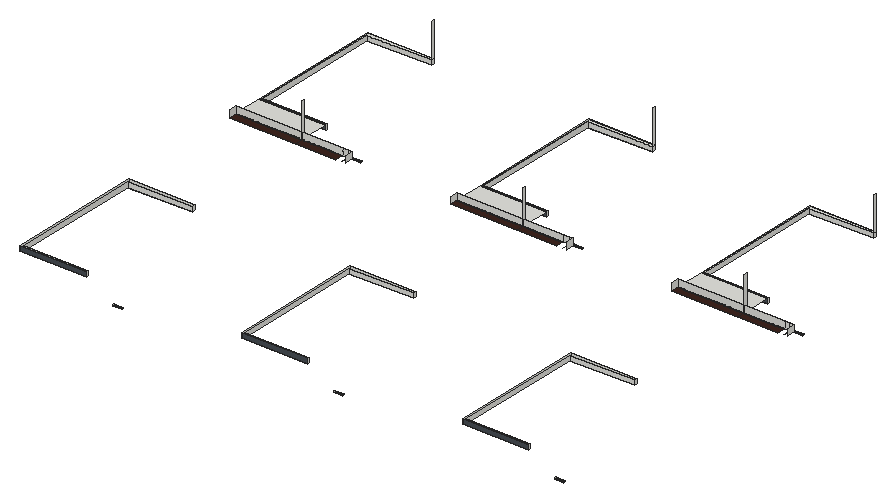
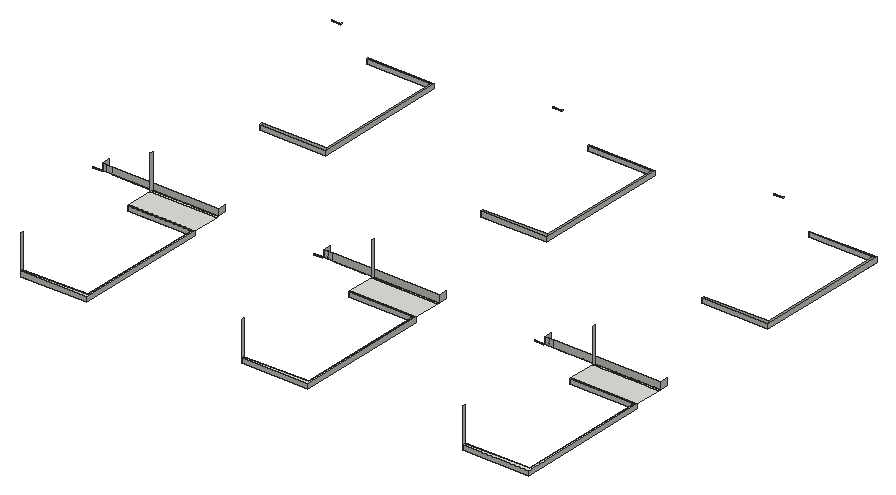
# SketchUp Ruby script. Lengths in inches.
U = 1.inch
M = Sketchup.active_model
def pt(a) = Geom::Point3d.new(a.map { |v| v * U })
def face(e, loops, mat)
  f = e.add_face(loops[0].map { |a| pt(a) })
  loops[1..].each { |l| e.add_face(l.map { |a| pt(a) }).erase! }
  f.material = f.back_material = mat if mat
  f
end
# faces: each face lists its corners as indices into pts; further lists are holes
def faces(e, pts, list, mat = nil) = list.each { |f| face(e, (f[0].is_a?(Array) ? f : [f]).map { |l| l.map { |i| pts[i] } }, mat) }
# xy, xz, yz: faces in a plane at the given z, y or x. An outline is a flat list of corners, or four numbers for a rectangle; further outlines are holes
def ring(l) = l.size == 4 ? [[l[0], l[1]], [l[2], l[1]], [l[2], l[3]], [l[0], l[3]]] : l.each_slice(2).to_a
def flat(e, list, mat, &to3) = list.each { |f| face(e, (f[0].is_a?(Array) ? f : [f]).map { |l| ring(l).map { |u, v| to3.(u, v) } }, mat) }
def xy(e, z, list, mat = nil) = flat(e, list, mat) { |x, y| [x, y, z] }
def xz(e, y, list, mat = nil) = flat(e, list, mat) { |x, z| [x, y, z] }
def yz(e, x, list, mat = nil) = flat(e, list, mat) { |y, z| [x, y, z] }
def lines(e, pts, list) = list.each { |a, b| e.add_line(pt(pts[a]), pt(pts[b])) }
# prism: a flat outline (further loops are holes) pulled along v
def prism(e, loops, v, mat = nil)
  f = face(e, loops, mat); d = Geom::Vector3d.new(v.map { |x| x * U })
  f.pushpull(f.normal.samedirection?(d) ? d.length : -d.length)
end
def box(e, o, s, mat = nil) = prism(e, [[o, [o[0] + s[0], o[1], o[2]], [o[0] + s[0], o[1] + s[1], o[2]], [o[0], o[1] + s[1], o[2]]]], [0, 0, s[2]], mat)
def at(x, y, z, deg = 0) = Geom::Transformation.translation(pt([x, y, z])) * Geom::Transformation.rotation(ORIGIN, Z_AXIS, deg.degrees)
def axes(o, x, y, z) = Geom::Transformation.new([*x, 0, *y, 0, *z, 0, *pt(o).to_a, 1])
def part(name) = M.definitions.add(name)
# library, detail: a bought-in or finely detailed component or shape, given as its bounding box
def library(name, o, s) = part(name).tap { |d| box(d.entities, o, s) }
def detail(e, o, s) = box(e.add_group.entities, o, s)
def put(e, d, t, mat = nil) = e.add_instance(d, t).tap { |i| i.material = mat if mat }
def group(e, t, mat = nil) = e.add_group.tap { |g| g.transformation = t; g.material = mat if mat }.entities
root = M.entities
M.materials.add("[0043_SaddleBrown]").color = [63, 38, 31]
M.materials.add("[Formica Blue]").color = [73, 80, 86]
xy(root,718,[[137.5,535.375,137.5,980.35,353.97,980.35,353.97,971.23,144.84,965.96,144.84,540.48,353.97,540.48,353.97,535.375],[861.9375,535.375,861.9375,980.35,1078.41,980.35,1078.41,971.23,869.28,965.96,869.28,540.48,1078.41,540.48,1078.41,535.375],[1586.375,535.375,1586.375,980.35,1802.84,980.35,1802.84,971.23,1593.72,965.96,1593.72,540.48,1802.84,540.48,1802.84,535.375],[137.5,1515.73,137.5,1960.7,353.97,1960.7,353.97,1951.58,144.84,1946.3125,144.84,1520.83,353.97,1520.83,353.97,1515.73],[861.9375,1515.73,861.9375,1960.7,1078.41,1960.7,1078.41,1951.58,869.28,1946.3125,869.28,1520.83,1078.41,1520.83,1078.41,1515.73],
  [1586.375,1515.73,1586.375,1960.7,1802.84,1960.7,1802.84,1951.58,1593.72,1946.3125,1593.72,1520.83,1802.84,1520.83,1802.84,1515.73]])
xy(root,733.125,[[517.3125,438.72,547.05,442.66],[1241.75,438.72,1271.49,442.66],[1966.1875,438.72,1995.93,442.66],[137.6,1417.45,139.16,1419.07],[139.16,1417.45,143.93,1419.07],
  [147.91,1417.45,149.47,1419.07],[149.47,1417.45,154.24,1419.07],[156.8,1417.45,158.36,1419.07],[158.36,1417.45,163.14,1419.07],[165.69,1417.45,167.25,1419.07],
  [167.25,1417.45,172.03,1419.07],[174.59,1417.45,176.14,1419.07],[176.14,1417.45,180.92,1419.07],[183.48,1417.45,185.03,1419.07],[185.03,1417.45,189.81,1419.07],
  [192.37,1417.45,193.92,1419.07],[193.92,1417.45,198.7,1419.07],[201.26,1417.45,202.82,1419.07],[202.82,1417.45,207.59,1419.07],[210.15,1417.45,211.71,1419.07],
  [211.71,1417.45,216.48,1419.07],[219.04,1417.45,220.6,1419.07],[220.6,1417.45,225.375,1419.07],[227.93,1417.45,229.49,1419.07],[229.49,1417.45,234.27,1419.07],
  [236.82,1417.45,238.38,1419.07],[238.38,1417.45,243.16,1419.07],[245.72,1417.45,247.27,1419.07],[247.27,1417.45,252.05,1419.07],[254.61,1417.45,256.16,1419.07],
  [256.16,1417.45,260.94,1419.07],[263.5,1417.45,265.05,1419.07],[265.05,1417.45,269.83,1419.07],[272.39,1417.45,273.95,1419.07],[273.95,1417.45,278.72,1419.07],
  [281.28,1417.45,282.84,1419.07],[282.84,1417.45,287.61,1419.07],[290.17,1417.45,291.73,1419.07],[291.73,1417.45,296.51,1419.07],[299.0625,1417.45,300.62,1419.07],
  [300.62,1417.45,305.4,1419.07],[307.95,1417.45,309.51,1419.07],[309.51,1417.45,314.29,1419.07],[316.85,1417.45,318.4,1419.07],[318.4,1417.45,323.18,1419.07],
  [325.74,1417.45,327.29,1419.07],[327.29,1417.45,332.07,1419.07],[334.63,1417.45,336.19,1419.07],[336.19,1417.45,340.96,1419.07],[343.52,1417.45,345.08,1419.07],
  [345.08,1417.45,349.85,1419.07],[352.41,1417.45,353.97,1419.07],[353.97,1417.45,358.74,1419.07],[361.3,1417.45,367.0625,1419.07],[369.3,1417.45,375.0625,1419.07],
  [377.3,1417.45,383.0625,1419.07],[385.3,1417.45,391.0625,1419.07],[393.3,1417.45,399.0625,1419.07],[401.3,1417.45,407.0625,1419.07],[409.3,1417.45,415.0625,1419.07],
  [417.3,1417.45,423.0625,1419.07],[425.3,1417.45,431.0625,1419.07],[433.3,1417.45,439.0625,1419.07],[441.3,1417.45,447.0625,1419.07],[449.3,1417.45,455.0625,1419.07],
  [457.3,1417.45,463.0625,1419.07],[862.04,1417.45,863.59,1419.07],[863.59,1417.45,868.37,1419.07],[872.35,1417.45,873.91,1419.07],[873.91,1417.45,878.68,1419.07],
  [881.24,1417.45,882.8,1419.07],[882.8,1417.45,887.57,1419.07],[890.13,1417.45,891.6875,1419.07],[891.6875,1417.45,896.47,1419.07],[899.02,1417.45,900.58,1419.07],
  [900.58,1417.45,905.36,1419.07],[907.91,1417.45,909.47,1419.07],[909.47,1417.45,914.25,1419.07],[916.81,1417.45,918.36,1419.07],[918.36,1417.45,923.14,1419.07],
  [925.7,1417.45,927.25,1419.07],[927.25,1417.45,932.03,1419.07],[934.59,1417.45,936.14,1419.07],[936.14,1417.45,940.92,1419.07],[943.48,1417.45,945.04,1419.07],
  [945.04,1417.45,949.8125,1419.07],[952.37,1417.45,953.93,1419.07],[953.93,1417.45,958.7,1419.07],[961.26,1417.45,962.82,1419.07],[962.82,1417.45,967.6,1419.07],
  [970.15,1417.45,971.71,1419.07],[971.71,1417.45,976.49,1419.07],[979.04,1417.45,980.6,1419.07],[980.6,1417.45,985.38,1419.07],[987.9375,1417.45,989.49,1419.07],
  [989.49,1417.45,994.27,1419.07],[996.83,1417.45,998.38,1419.07],[998.38,1417.45,1003.16,1419.07],[1005.72,1417.45,1007.27,1419.07],[1007.27,1417.45,1012.05,1419.07],
  [1014.61,1417.45,1016.17,1419.07],[1016.17,1417.45,1020.94,1419.07],[1023.5,1417.45,1025.06,1419.07],[1025.06,1417.45,1029.83,1419.07],[1032.39,1417.45,1033.95,1419.07],
  [1033.95,1417.45,1038.73,1419.07],[1041.28,1417.45,1042.84,1419.07],[1042.84,1417.45,1047.62,1419.07],[1050.17,1417.45,1051.73,1419.07],[1051.73,1417.45,1056.51,1419.07],
  [1059.07,1417.45,1060.62,1419.07],[1060.62,1417.45,1065.4,1419.07],[1067.96,1417.45,1069.51,1419.07],[1069.51,1417.45,1074.29,1419.07],[1076.85,1417.45,1078.41,1419.07],
  [1078.41,1417.45,1083.18,1419.07],[1085.74,1417.45,1091.5,1419.07],[1093.74,1417.45,1099.5,1419.07],[1101.74,1417.45,1107.5,1419.07],[1109.74,1417.45,1115.5,1419.07],
  [1117.74,1417.45,1123.5,1419.07],[1125.74,1417.45,1131.5,1419.07],[1133.74,1417.45,1139.5,1419.07],[1141.74,1417.45,1147.5,1419.07],[1149.74,1417.45,1155.5,1419.07],
  [1157.74,1417.45,1163.5,1419.07],[1165.74,1417.45,1171.5,1419.07],[1173.74,1417.45,1179.5,1419.07],[1181.74,1417.45,1187.5,1419.07],[1189.74,1417.45,1195.5,1419.07],
  [1197.74,1417.45,1203.5,1419.07],[1205.74,1417.45,1211.5,1419.07],[1586.47,1417.45,1588.03,1419.07],[1588.03,1417.45,1592.81,1419.07],[1596.79,1417.45,1598.34,1419.07],
  [1598.34,1417.45,1603.12,1419.07],[1605.68,1417.45,1607.23,1419.07],[1607.23,1417.45,1612.01,1419.07],[1614.57,1417.45,1616.125,1419.07],[1616.125,1417.45,1620.9,1419.07],
  [1623.46,1417.45,1625.02,1419.07],[1625.02,1417.45,1629.79,1419.07],[1632.35,1417.45,1633.91,1419.07],[1633.91,1417.45,1638.69,1419.07],[1641.24,1417.45,1642.8,1419.07],
  [1642.8,1417.45,1647.58,1419.07],[1650.13,1417.45,1651.69,1419.07],[1651.69,1417.45,1656.47,1419.07],[1659.03,1417.45,1660.58,1419.07],[1660.58,1417.45,1665.36,1419.07],
  [1667.92,1417.45,1669.47,1419.07],[1669.47,1417.45,1674.25,1419.07],[1676.81,1417.45,1678.36,1419.07],[1678.36,1417.45,1683.14,1419.07],[1685.7,1417.45,1687.26,1419.07],
  [1687.26,1417.45,1692.03,1419.07],[1694.59,1417.45,1696.15,1419.07],[1696.15,1417.45,1700.92,1419.07],[1703.48,1417.45,1705.04,1419.07],[1705.04,1417.45,1709.82,1419.07],
  [1712.375,1417.45,1713.93,1419.07],[1713.93,1417.45,1718.71,1419.07],[1721.26,1417.45,1722.82,1419.07],[1722.82,1417.45,1727.6,1419.07],[1730.16,1417.45,1731.71,1419.07],
  [1731.71,1417.45,1736.49,1419.07],[1739.05,1417.45,1740.6,1419.07],[1740.6,1417.45,1745.38,1419.07],[1747.9375,1417.45,1749.5,1419.07],[1749.5,1417.45,1754.27,1419.07],
  [1756.83,1417.45,1758.39,1419.07],[1758.39,1417.45,1763.16,1419.07],[1765.72,1417.45,1767.28,1419.07],[1767.28,1417.45,1772.05,1419.07],[1774.61,1417.45,1776.17,1419.07],
  [1776.17,1417.45,1780.95,1419.07],[1783.5,1417.45,1785.06,1419.07],[1785.06,1417.45,1789.84,1419.07],[1792.39,1417.45,1793.95,1419.07],[1793.95,1417.45,1798.73,1419.07],
  [1801.29,1417.45,1802.84,1419.07],[1802.84,1417.45,1807.62,1419.07],[1810.18,1417.45,1815.9375,1419.07],[1818.18,1417.45,1823.9375,1419.07],[1826.18,1417.45,1831.9375,1419.07],
  [1834.18,1417.45,1839.9375,1419.07],[1842.18,1417.45,1847.9375,1419.07],[1850.18,1417.45,1855.9375,1419.07],[1858.18,1417.45,1863.9375,1419.07],[1866.18,1417.45,1871.9375,1419.07],
  [1874.18,1417.45,1879.9375,1419.07],[1882.18,1417.45,1887.9375,1419.07],[1890.18,1417.45,1895.9375,1419.07],[1898.18,1417.45,1903.9375,1419.07],[1906.18,1417.45,1911.9375,1419.07],
  [1914.18,1417.45,1919.9375,1419.07],[1922.18,1417.45,1927.9375,1419.07],[1930.18,1417.45,1935.9375,1419.07],[137.5,1419.07,353.97,1428.19],[517.3125,1419.07,547.05,1423.01],
  [861.9375,1419.07,1078.41,1428.19],[1241.75,1419.07,1271.49,1423.01],[1586.375,1419.07,1802.84,1428.19],[1966.1875,1419.07,1995.93,1423.01],[137.5,1428.19,353.97,1515.73],
  [861.9375,1428.19,1078.41,1515.73],[1586.375,1428.19,1802.84,1515.73],[137.5,1515.73,353.97,1515.73,353.97,1520.83,144.84,1520.83,144.84,1946.3125,353.97,1951.58,353.97,1960.7,137.5,1960.7],[861.9375,1515.73,1078.41,1515.73,1078.41,1520.83,869.28,1520.83,869.28,1946.3125,1078.41,1951.58,1078.41,1960.7,861.9375,1960.7],[1586.375,1515.73,1802.84,1515.73,1802.84,1520.83,1593.72,1520.83,1593.72,1946.3125,1802.84,1951.58,1802.84,1960.7,1586.375,1960.7]])
xy(root,733.125,[[137.5,1392.39,353.97,1392.39,353.97,1417.45,352.41,1417.45,352.41,1419.07,349.85,1419.07,349.85,1417.45,343.52,1417.45,343.52,1419.07,340.96,1419.07,340.96,1417.45,334.63,1417.45,334.63,1419.07,332.07,1419.07,332.07,1417.45,325.74,1417.45,325.74,1419.07,323.18,1419.07,323.18,1417.45,316.85,1417.45,316.85,1419.07,314.29,1419.07,314.29,1417.45,307.95,1417.45,307.95,1419.07,305.4,1419.07,305.4,1417.45,299.0625,1417.45,299.0625,1419.07,296.51,1419.07,296.51,1417.45,290.17,1417.45,290.17,1419.07,287.61,1419.07,287.61,1417.45,281.28,1417.45,281.28,1419.07,278.72,1419.07,278.72,1417.45,272.39,1417.45,272.39,1419.07,269.83,1419.07,269.83,1417.45,263.5,1417.45,263.5,1419.07,260.94,1419.07,260.94,1417.45,254.61,1417.45,254.61,1419.07,252.05,1419.07,252.05,1417.45,245.72,1417.45,245.72,1419.07,243.16,1419.07,243.16,1417.45,236.82,1417.45,236.82,1419.07,234.27,1419.07,234.27,1417.45,227.93,1417.45,227.93,1419.07,225.375,1419.07,225.375,1417.45,219.04,1417.45,219.04,1419.07,216.48,1419.07,216.48,1417.45,210.15,1417.45,210.15,1419.07,207.59,1419.07,207.59,1417.45,201.26,1417.45,201.26,1419.07,198.7,1419.07,198.7,1417.45,192.37,1417.45,192.37,1419.07,189.81,1419.07,189.81,1417.45,183.48,1417.45,183.48,1419.07,180.92,1419.07,180.92,1417.45,174.59,1417.45,174.59,1419.07,172.03,1419.07,172.03,1417.45,165.69,1417.45,165.69,1419.07,163.14,1419.07,163.14,1417.45,156.8,1417.45,156.8,1419.07,154.24,1419.07,154.24,1417.45,147.91,1417.45,147.91,1419.07,143.93,1419.07,143.93,1417.45,137.6,1417.45,137.6,1419.07,137.5,1419.07],[353.97,1392.39,353.97,1417.45,358.74,1417.45,358.74,1419.07,361.3,1419.07,361.3,1417.45,367.0625,1417.45,367.0625,1419.07,369.3,1419.07,369.3,1417.45,375.0625,1417.45,375.0625,1419.07,377.3,1419.07,377.3,1417.45,383.0625,1417.45,383.0625,1419.07,385.3,1419.07,385.3,1417.45,391.0625,1417.45,391.0625,1419.07,393.3,1419.07,393.3,1417.45,399.0625,1417.45,399.0625,1419.07,401.3,1419.07,401.3,1417.45,407.0625,1417.45,407.0625,1419.07,409.3,1419.07,409.3,1417.45,415.0625,1417.45,415.0625,1419.07,417.3,1419.07,417.3,1417.45,423.0625,1417.45,423.0625,1419.07,425.3,1419.07,425.3,1417.45,431.0625,1417.45,431.0625,1419.07,433.3,1419.07,433.3,1417.45,439.0625,1417.45,439.0625,1419.07,441.3,1419.07,441.3,1417.45,447.0625,1417.45,447.0625,1419.07,449.3,1419.07,449.3,1417.45,455.0625,1417.45,455.0625,1419.07,457.3,1419.07,457.3,1417.45,463.0625,1417.45,463.0625,1419.07,465.3,1419.07,465.3,1417.45,471.0625,1417.45,471.0625,1419.07,473.3,1419.07,473.3,1417.45,479.0625,1417.45,479.0625,1419.07,481.3,1419.07,481.3,1417.45,487.0625,1417.45,487.0625,1392.39],[861.9375,1392.39,1078.41,1392.39,1078.41,1417.45,1076.85,1417.45,1076.85,1419.07,1074.29,1419.07,1074.29,1417.45,1067.96,1417.45,1067.96,1419.07,1065.4,1419.07,1065.4,1417.45,1059.07,1417.45,1059.07,1419.07,1056.51,1419.07,1056.51,1417.45,1050.17,1417.45,1050.17,1419.07,1047.62,1419.07,1047.62,1417.45,1041.28,1417.45,1041.28,1419.07,1038.73,1419.07,1038.73,1417.45,1032.39,1417.45,1032.39,1419.07,1029.83,1419.07,1029.83,1417.45,1023.5,1417.45,1023.5,1419.07,1020.94,1419.07,1020.94,1417.45,1014.61,1417.45,1014.61,1419.07,1012.05,1419.07,1012.05,1417.45,1005.72,1417.45,1005.72,1419.07,1003.16,1419.07,1003.16,1417.45,996.83,1417.45,996.83,1419.07,994.27,1419.07,994.27,1417.45,987.9375,1417.45,987.9375,1419.07,985.38,1419.07,985.38,1417.45,979.04,1417.45,979.04,1419.07,976.49,1419.07,976.49,1417.45,970.15,1417.45,970.15,1419.07,967.6,1419.07,967.6,1417.45,961.26,1417.45,961.26,1419.07,958.7,1419.07,958.7,1417.45,952.37,1417.45,952.37,1419.07,949.8125,1419.07,949.8125,1417.45,943.48,1417.45,943.48,1419.07,940.92,1419.07,940.92,1417.45,934.59,1417.45,934.59,1419.07,932.03,1419.07,932.03,1417.45,925.7,1417.45,925.7,1419.07,923.14,1419.07,923.14,1417.45,916.81,1417.45,916.81,1419.07,914.25,1419.07,914.25,1417.45,907.91,1417.45,907.91,1419.07,905.36,1419.07,905.36,1417.45,899.02,1417.45,899.02,1419.07,896.47,1419.07,896.47,1417.45,890.13,1417.45,890.13,1419.07,887.57,1419.07,887.57,1417.45,881.24,1417.45,881.24,1419.07,878.68,1419.07,878.68,1417.45,872.35,1417.45,872.35,1419.07,868.37,1419.07,868.37,1417.45,862.04,1417.45,862.04,1419.07,861.9375,1419.07],[1078.41,1392.39,1078.41,1417.45,1083.18,1417.45,1083.18,1419.07,1085.74,1419.07,1085.74,1417.45,1091.5,1417.45,1091.5,1419.07,1093.74,1419.07,1093.74,1417.45,1099.5,1417.45,1099.5,1419.07,1101.74,1419.07,1101.74,1417.45,1107.5,1417.45,1107.5,1419.07,1109.74,1419.07,1109.74,1417.45,1115.5,1417.45,1115.5,1419.07,1117.74,1419.07,1117.74,1417.45,1123.5,1417.45,1123.5,1419.07,1125.74,1419.07,1125.74,1417.45,1131.5,1417.45,1131.5,1419.07,1133.74,1419.07,1133.74,1417.45,1139.5,1417.45,1139.5,1419.07,1141.74,1419.07,1141.74,1417.45,1147.5,1417.45,1147.5,1419.07,1149.74,1419.07,1149.74,1417.45,1155.5,1417.45,1155.5,1419.07,1157.74,1419.07,1157.74,1417.45,1163.5,1417.45,1163.5,1419.07,1165.74,1419.07,1165.74,1417.45,1171.5,1417.45,1171.5,1419.07,1173.74,1419.07,1173.74,1417.45,1179.5,1417.45,1179.5,1419.07,1181.74,1419.07,1181.74,1417.45,1187.5,1417.45,1187.5,1419.07,1189.74,1419.07,1189.74,1417.45,1195.5,1417.45,1195.5,1419.07,1197.74,1419.07,1197.74,1417.45,1203.5,1417.45,1203.5,1419.07,1205.74,1419.07,1205.74,1417.45,1211.5,1417.45,1211.5,1392.39],[1586.375,1392.39,1802.84,1392.39,1802.84,1417.45,1801.29,1417.45,1801.29,1419.07,1798.73,1419.07,1798.73,1417.45,1792.39,1417.45,1792.39,1419.07,1789.84,1419.07,1789.84,1417.45,1783.5,1417.45,1783.5,1419.07,1780.95,1419.07,1780.95,1417.45,1774.61,1417.45,1774.61,1419.07,1772.05,1419.07,1772.05,1417.45,1765.72,1417.45,1765.72,1419.07,1763.16,1419.07,1763.16,1417.45,1756.83,1417.45,1756.83,1419.07,1754.27,1419.07,1754.27,1417.45,1747.9375,1417.45,1747.9375,1419.07,1745.38,1419.07,1745.38,1417.45,1739.05,1417.45,1739.05,1419.07,1736.49,1419.07,1736.49,1417.45,1730.16,1417.45,1730.16,1419.07,1727.6,1419.07,1727.6,1417.45,1721.26,1417.45,1721.26,1419.07,1718.71,1419.07,1718.71,1417.45,1712.375,1417.45,1712.375,1419.07,1709.82,1419.07,1709.82,1417.45,1703.48,1417.45,1703.48,1419.07,1700.92,1419.07,1700.92,1417.45,1694.59,1417.45,1694.59,1419.07,1692.03,1419.07,1692.03,1417.45,1685.7,1417.45,1685.7,1419.07,1683.14,1419.07,1683.14,1417.45,1676.81,1417.45,1676.81,1419.07,1674.25,1419.07,1674.25,1417.45,1667.92,1417.45,1667.92,1419.07,1665.36,1419.07,1665.36,1417.45,1659.03,1417.45,1659.03,1419.07,1656.47,1419.07,1656.47,1417.45,1650.13,1417.45,1650.13,1419.07,1647.58,1419.07,1647.58,1417.45,1641.24,1417.45,1641.24,1419.07,1638.69,1419.07,1638.69,1417.45,1632.35,1417.45,1632.35,1419.07,1629.79,1419.07,1629.79,1417.45,1623.46,1417.45,1623.46,1419.07,1620.9,1419.07,1620.9,1417.45,1614.57,1417.45,1614.57,1419.07,1612.01,1419.07,1612.01,1417.45,1605.68,1417.45,1605.68,1419.07,1603.12,1419.07,1603.12,1417.45,1596.79,1417.45,1596.79,1419.07,1592.81,1419.07,1592.81,1417.45,1586.47,1417.45,1586.47,1419.07,1586.375,1419.07],
  [1802.84,1392.39,1802.84,1417.45,1807.62,1417.45,1807.62,1419.07,1810.18,1419.07,1810.18,1417.45,1815.9375,1417.45,1815.9375,1419.07,1818.18,1419.07,1818.18,1417.45,1823.9375,1417.45,1823.9375,1419.07,1826.18,1419.07,1826.18,1417.45,1831.9375,1417.45,1831.9375,1419.07,1834.18,1419.07,1834.18,1417.45,1839.9375,1417.45,1839.9375,1419.07,1842.18,1419.07,1842.18,1417.45,1847.9375,1417.45,1847.9375,1419.07,1850.18,1419.07,1850.18,1417.45,1855.9375,1417.45,1855.9375,1419.07,1858.18,1419.07,1858.18,1417.45,1863.9375,1417.45,1863.9375,1419.07,1866.18,1419.07,1866.18,1417.45,1871.9375,1417.45,1871.9375,1419.07,1874.18,1419.07,1874.18,1417.45,1879.9375,1417.45,1879.9375,1419.07,1882.18,1419.07,1882.18,1417.45,1887.9375,1417.45,1887.9375,1419.07,1890.18,1419.07,1890.18,1417.45,1895.9375,1417.45,1895.9375,1419.07,1898.18,1419.07,1898.18,1417.45,1903.9375,1417.45,1903.9375,1419.07,1906.18,1419.07,1906.18,1417.45,1911.9375,1417.45,1911.9375,1419.07,1914.18,1419.07,1914.18,1417.45,1919.9375,1417.45,1919.9375,1419.07,1922.18,1419.07,1922.18,1417.45,1927.9375,1417.45,1927.9375,1419.07,1930.18,1419.07,1930.18,1417.45,1935.9375,1417.45,1935.9375,1392.39]],"[0043_SaddleBrown]")
xz(root,442.66,[[517.3125,733.125,547.05,736],[1241.75,733.125,1271.49,736],[1966.1875,733.125,1995.93,736]],"[0043_SaddleBrown]")
xz(root,535.375,[[137.5,718,353.97,733.125],[861.9375,718,1078.41,733.125],[1586.375,718,1802.84,733.125]],"[Formica Blue]")
xz(root,540.48,[[144.84,718,353.97,733.125],[869.28,718,1078.41,733.125],[1593.72,718,1802.84,733.125]])
xz(root,980.35,[[137.5,718,353.97,733.125],[861.9375,718,1078.41,733.125],[1586.375,718,1802.84,733.125]])
xz(root,1419.07,[[137.5,733.125,353.97,755.5],[353.97,733.125,487.0625,755.5],[487.0625,733.125,504.5,755.5],[504.5,733.125,517.3125,755.5],[861.9375,733.125,1078.41,755.5],
  [1078.41,733.125,1211.5,755.5],[1211.5,733.125,1228.9375,755.5],[1228.9375,733.125,1241.75,755.5],[1586.375,733.125,1802.84,755.5],[1802.84,733.125,1935.9375,755.5],
  [1935.9375,733.125,1953.375,755.5],[1953.375,733.125,1966.1875,755.5]])
xz(root,1423.01,[[517.3125,733.125,547.05,736],[1241.75,733.125,1271.49,736],[1966.1875,733.125,1995.93,736]],"[0043_SaddleBrown]")
xz(root,1515.73,[[137.5,718,353.97,733.125],[861.9375,718,1078.41,733.125],[1586.375,718,1802.84,733.125]],"[Formica Blue]")
xz(root,1520.83,[[144.84,718,353.97,733.125],[869.28,718,1078.41,733.125],[1593.72,718,1802.84,733.125]])
xz(root,1960.7,[[137.5,718,353.97,733.125],[861.9375,718,1078.41,733.125],[1586.375,718,1802.84,733.125]])
yz(root,137.5,[[535.375,718,980.35,733.125],[1515.73,718,1960.7,733.125],[1392.39,733.125,1419.07,755.5]])
yz(root,144.84,[[540.48,718,965.96,733.125],[1520.83,718,1946.3125,733.125]])
yz(root,353.97,[[535.375,718,540.48,733.125],[971.23,718,980.35,733.125],[1515.73,718,1520.83,733.125],[1951.58,718,1960.7,733.125],[1419.07,733.125,1428.19,845.41],
  [1951.58,733.125,1960.7,845.41]])
yz(root,517.3125,[[438.72,733.125,442.66,736],[1392.39,733.125,1419.07,755.5],[1419.07,733.125,1423.01,736]])
yz(root,861.9375,[[535.375,718,980.35,733.125],[1515.73,718,1960.7,733.125],[1392.39,733.125,1419.07,755.5]])
yz(root,869.28,[[540.48,718,965.96,733.125],[1520.83,718,1946.3125,733.125]])
yz(root,1078.41,[[535.375,718,540.48,733.125],[971.23,718,980.35,733.125],[1515.73,718,1520.83,733.125],[1951.58,718,1960.7,733.125],[1419.07,733.125,1428.19,845.41],
  [1951.58,733.125,1960.7,845.41]])
yz(root,1241.75,[[438.72,733.125,442.66,736],[1392.39,733.125,1419.07,755.5],[1419.07,733.125,1423.01,736]])
yz(root,1586.375,[[535.375,718,980.35,733.125],[1515.73,718,1960.7,733.125],[1392.39,733.125,1419.07,755.5]])
yz(root,1593.72,[[540.48,718,965.96,733.125],[1520.83,718,1946.3125,733.125]])
yz(root,1802.84,[[535.375,718,540.48,733.125],[971.23,718,980.35,733.125],[1515.73,718,1520.83,733.125],[1951.58,718,1960.7,733.125],[1419.07,733.125,1428.19,845.41],
  [1951.58,733.125,1960.7,845.41]])
yz(root,1966.1875,[[438.72,733.125,442.66,736],[1392.39,733.125,1419.07,755.5],[1419.07,733.125,1423.01,736]])
p = [[144.84,965.96,718],[353.97,971.23,718],[353.97,971.23,733.125],[144.84,965.96,733.125],[869.28,965.96,718],[1078.41,971.23,718],
  [1078.41,971.23,733.125],[869.28,965.96,733.125],[1593.72,965.96,718],[1802.84,971.23,718],[1802.84,971.23,733.125],[1593.72,965.96,733.125],
  [144.84,1946.3125,718],[353.97,1951.58,718],[353.97,1951.58,733.125],[144.84,1946.3125,733.125],[869.28,1946.3125,718],[1078.41,1951.58,718],
  [1078.41,1951.58,733.125],[869.28,1946.3125,733.125],[1593.72,1946.3125,718],[1802.84,1951.58,718],[1802.84,1951.58,733.125],[1593.72,1946.3125,733.125],
  [1228.9375,1419.07,733.125],[1228.9375,1392.39,733.125],[1953.375,1419.07,733.125],[1953.375,1392.39,733.125],[504.5,1419.07,733.125],[504.5,1392.39,733.125]]
faces(root,p,[[0,1,2,3],[4,5,6,7],[8,9,10,11],[12,13,14,15],[16,17,18,19],[20,21,22,23]])
lines(root,p,[[24,25],[26,27],[28,29]])
